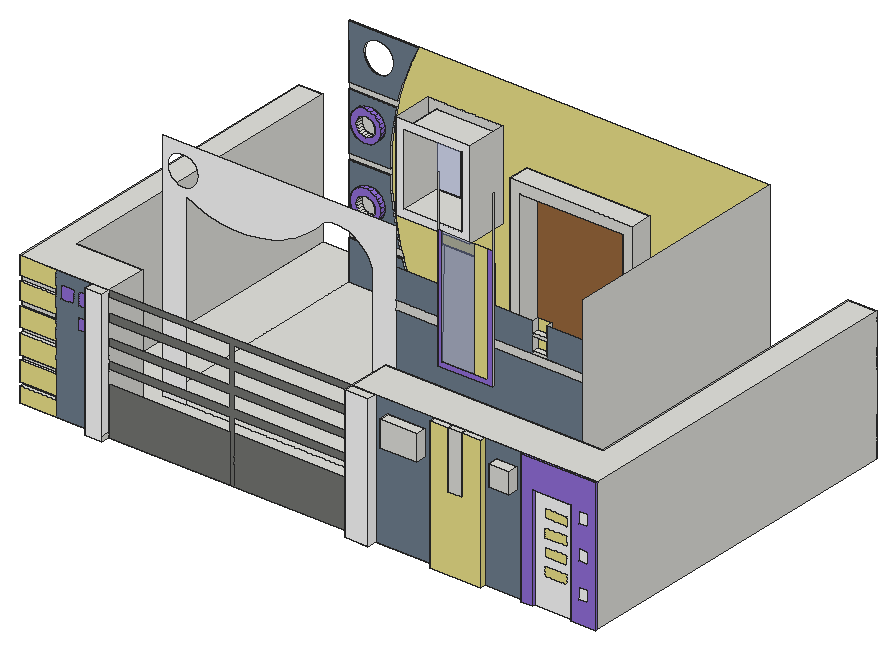
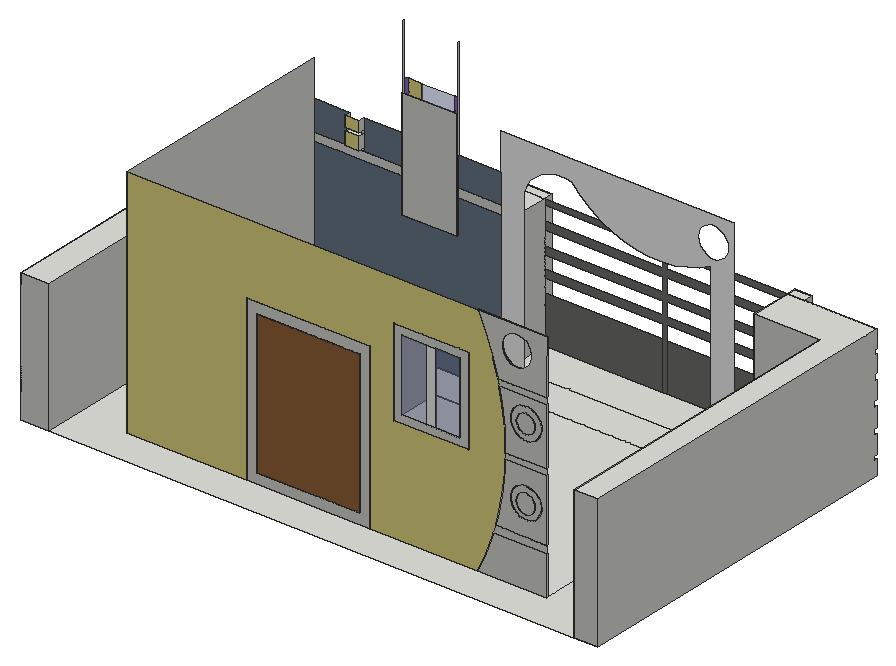
# SketchUp Ruby script. Lengths in inches.
U = 1.inch
M = Sketchup.active_model
def pt(a) = Geom::Point3d.new(a.map { |v| v * U })
def face(e, loops, mat)
  f = e.add_face(loops[0].map { |a| pt(a) })
  loops[1..].each { |l| e.add_face(l.map { |a| pt(a) }).erase! }
  f.material = f.back_material = mat if mat
  f
end
# faces: each face lists its corners as indices into pts; further lists are holes
def faces(e, pts, list, mat = nil) = list.each { |f| face(e, (f[0].is_a?(Array) ? f : [f]).map { |l| l.map { |i| pts[i] } }, mat) }
# xy, xz, yz: faces in a plane at the given z, y or x. An outline is a flat list of corners, or four numbers for a rectangle; further outlines are holes
def ring(l) = l.size == 4 ? [[l[0], l[1]], [l[2], l[1]], [l[2], l[3]], [l[0], l[3]]] : l.each_slice(2).to_a
def flat(e, list, mat, &to3) = list.each { |f| face(e, (f[0].is_a?(Array) ? f : [f]).map { |l| ring(l).map { |u, v| to3.(u, v) } }, mat) }
def xy(e, z, list, mat = nil) = flat(e, list, mat) { |x, y| [x, y, z] }
def xz(e, y, list, mat = nil) = flat(e, list, mat) { |x, z| [x, y, z] }
def yz(e, x, list, mat = nil) = flat(e, list, mat) { |y, z| [x, y, z] }
def lines(e, pts, list) = list.each { |a, b| e.add_line(pt(pts[a]), pt(pts[b])) }
# prism: a flat outline (further loops are holes) pulled along v
def prism(e, loops, v, mat = nil)
  f = face(e, loops, mat); d = Geom::Vector3d.new(v.map { |x| x * U })
  f.pushpull(f.normal.samedirection?(d) ? d.length : -d.length)
end
def box(e, o, s, mat = nil) = prism(e, [[o, [o[0] + s[0], o[1], o[2]], [o[0] + s[0], o[1] + s[1], o[2]], [o[0], o[1] + s[1], o[2]]]], [0, 0, s[2]], mat)
def at(x, y, z, deg = 0) = Geom::Transformation.translation(pt([x, y, z])) * Geom::Transformation.rotation(ORIGIN, Z_AXIS, deg.degrees)
def axes(o, x, y, z) = Geom::Transformation.new([*x, 0, *y, 0, *z, 0, *pt(o).to_a, 1])
def part(name) = M.definitions.add(name)
# library, detail: a bought-in or finely detailed component or shape, given as its bounding box
def library(name, o, s) = part(name).tap { |d| box(d.entities, o, s) }
def detail(e, o, s) = box(e.add_group.entities, o, s)
def put(e, d, t, mat = nil) = e.add_instance(d, t).tap { |i| i.material = mat if mat }
def group(e, t, mat = nil) = e.add_group.tap { |g| g.transformation = t; g.material = mat if mat }.entities
root = M.entities
M.materials.add("[0047_Khaki]").color = [240, 230, 140]
M.materials.add("[0111_SlateGray]").color = [112, 128, 144]
M.materials.add("[0115_MediumPurple]").color = [147, 112, 219]
M.materials.add("[0128_White]").color = [255, 255, 255]
M.materials.add("[Metal Seamed]").color = [118, 119, 115]
M.materials.add("[Translucent Glass Sky Reflection]").color = [126, 138, 183]
M.materials["[Translucent Glass Sky Reflection]"].alpha = 0.52
M.materials.add("[Wood Floor]").color = [155, 105, 61]
xy(root,0,[[36.78,0.6875,45.64,5.3125],[170.23,0.6875,182.3125,5.3125],[212.8,2.1875,238.66,5.3125],[258.03,3.6875,264.32,5.3125],[283.76,3.6875,296.5,5.3125],
  [0,5.3125,0,184,12.1,184,12.1,26.76,45.64,26.76,45.64,5.3125],[45.64,5.3125,170.23,26.76],[170.23,5.3125,170.23,26.76,282.06,26.76,282.06,184,296.5,184,296.5,5.3125],[[12.1,26.76,282.06,184],[40.75,45.625,256.75,165.625]],[40.75,45.625,40.75,164.9375,76.51,164.9375,76.51,165.625,131.6875,165.625,131.6875,154.6875,195,154.6875,195,165.625,256.75,165.625,256.75,45.625],
  [131.6875,154.6875,195,165.625],[40.75,164.9375,76.51,165.625]])
xy(root,5.41,[[137.1,154.6875,189.59,165.625]])
xy(root,7.86,[[0,5.3125,18.39,7.0625]])
xy(root,9.82,[[0,5.3125,18.39,7.0625]])
xy(root,19.55,[[0,5.3125,18.39,7.0625]])
xy(root,20.15,[[40.75,164.9375,68.39,165.625]])
xy(root,22.18,[[0,5.3125,18.39,7.0625]])
xy(root,24.17,[[40.75,164.9375,67.27,165.625]])
xy(root,32.3,[[0,5.3125,18.39,7.0625]])
xy(root,34.95,[[0,5.3125,18.39,7.0625]])
xy(root,38.3125,[[222.1,2.1875,228.92,5.3125]])
xy(root,44.42,[[0,5.3125,18.39,6.5]])
xy(root,47.25,[[0,5.3125,18.39,6.5]])
xy(root,47.92,[[188.84,0,207.78,5.3125]])
xy(root,49.69,[[244.53,0,255.09,5.3125]])
xy(root,53.625,[[264.32,3.6875,283.76,5.3125]],"[0115_MediumPurple]")
xy(root,53.875,[[81.125,144.5625,119.5625,165.625]])
xy(root,56.15,[[40.75,164.9375,62.41,165.625]])
xy(root,56.2,[[0,5.3125,18.39,6.5]])
xy(root,58.08,[[85.33,144.5625,115.36,165.625]])
xy(root,58.65,[[0,5.3125,18.39,6.5]])
xy(root,59.3125,[[40.75,164.9375,62.29,165.625]])
xy(root,60.25,[[244.53,0,255.09,5.3125]])
xy(root,61.11,[[188.84,0,207.78,5.3125]])
xy(root,64,[[182.75,44.5625,211.0625,45.625],[182.75,45.625,211.0625,45.9375]])
xy(root,67.8125,[[36.78,0.6875,45.64,5.3125],[170.23,0.6875,182.3125,5.3125],[212.8,2.1875,222.1,5.3125],[222.1,2.1875,228.92,5.3125],[228.92,2.1875,238.66,5.3125],
  [0,5.3125,45.64,5.3125,45.64,26.76,12.1,26.76,12.1,184,0,184],[170.23,5.3125,296.5,5.3125,296.5,184,282.06,184,282.06,26.76,170.23,26.76]])
xy(root,67.8125,[[258.03,3.6875,296.5,5.3125]],"[0115_MediumPurple]")
xy(root,78.59,[[137.1,154.6875,189.59,165.625]])
xy(root,84,[[131.6875,154.6875,195,165.625]])
xy(root,87.45,[[231.02,45.625,238.14,48.4375]])
xy(root,88.75,[[40.75,164.9375,65.47,165.625]])
xy(root,92.01,[[40.75,164.9375,66.2,165.625]])
xy(root,94.06,[[231.02,45.625,238.14,48.4375]])
xy(root,94.79,[[85.33,144.5625,115.36,165.625]])
xy(root,95.79,[[231.02,45.625,238.14,48.4375]])
xz(root,0,[[188.84,47.92,207.78,61.11],[244.53,49.69,255.09,60.25]])
xz(root,0.6875,[[36.78,0,45.64,67.8125],[170.23,0,182.3125,67.8125]],"[0128_White]")
xz(root,2.1875,[[222.1,38.3125,228.92,67.8125]])
xz(root,2.1875,[[212.8,0,238.66,0,238.66,67.8125,228.92,67.8125,228.92,38.3125,222.1,38.3125,222.1,67.8125,212.8,67.8125]],"[0047_Khaki]")
xz(root,3.6875,[[[258.03,0,264.32,0,264.32,53.625,283.76,53.625,283.76,0,296.5,0,296.5,67.8125,258.03,67.8125],[288.18,46.25,292.5,52.25],[288.18,29.0625,292.5,35.0625],[288.18,11.5,292.5,17.5]]],"[0115_MediumPurple]")
xz(root,3.6875,[[288.18,11.5,292.5,17.5],[288.18,29.0625,292.5,35.0625],[288.18,46.25,292.5,52.25]],"[0128_White]")
xz(root,5.3125,[[36.78,0,45.64,67.8125],[170.23,0,182.3125,67.8125],[212.8,0,212.8,67.8125,222.1,67.8125,222.1,38.3125,228.92,38.3125,228.92,67.8125,238.66,67.8125,238.66,0],[258.03,0,258.03,67.8125,296.5,67.8125,296.5,0,283.76,0,283.76,53.625,264.32,53.625,264.32,0],[222.1,38.3125,228.92,67.8125],
  [188.84,47.92,207.78,61.11],[244.53,49.69,255.09,60.25]])
xz(root,5.3125,[[0,0,18.39,7.86],[0,9.82,18.39,19.55],[269.1,14.74,280.41,19.43],[0,22.18,18.39,32.3],[269.1,23.68,280.41,28.37],
  [269.1,32.49,280.41,37.18],[0,34.95,18.39,44.42],[269.1,41.55,280.41,46.24],[0,47.25,18.39,56.2],[0,58.65,18.39,67.8125]],"[0047_Khaki]")
xz(root,5.3125,[[[18.39,0,36.78,67.8125],[20.96,55.08,27.39,61.52],[30.26,55.24,35.57,61.74],[30.26,44.17,35.95,49.85]],[[182.3125,0,212.8,67.8125],[188.84,47.92,207.78,61.11]],[[238.66,0,258.03,67.8125],[244.53,49.69,255.09,60.25]]],"[0111_SlateGray]")
xz(root,5.3125,[[30.26,44.17,35.95,49.85],[20.96,55.08,27.39,61.52],[30.26,55.24,35.57,61.74]],"[0115_MediumPurple]")
xz(root,5.3125,[[[264.32,0,283.76,53.625],[269.1,41.55,280.41,46.24],[269.1,32.49,280.41,37.18],[269.1,23.68,280.41,28.37],[269.1,14.74,280.41,19.43]]],"[0128_White]")
xz(root,5.3125,[[107.64,0,107.64,31.52,45.64,31.52,45.64,35.5,107.64,35.5,107.64,42.12,45.64,42.12,45.64,46.09,107.64,46.09,107.64,53.36,45.64,53.36,45.64,57.36,107.64,57.36,107.64,64.74,45.64,64.74,45.64,67.8125,170.23,67.8125,170.23,64.74,109.53,64.74,109.53,57.36,170.23,57.36,170.23,53.36,109.53,53.36,109.53,46.09,170.23,46.09,170.23,42.12,109.53,42.12,109.53,35.5,170.23,35.5,170.23,31.52,109.53,31.52,109.53,0],[45.64,0,107.64,24.54],[109.53,0,170.23,24.54]],"[Metal Seamed]")
xz(root,6.5,[[0,44.42,18.39,47.25],[0,56.2,18.39,58.65]])
xz(root,7.0625,[[0,7.86,18.39,9.82],[0,19.55,18.39,22.18],[0,32.3,18.39,34.95]])
xz(root,26.76,[[12.1,0,45.64,67.8125],[170.23,0,282.06,67.8125]])
xz(root,44.5625,[[201.68,66.53,208.37,66.53,208.5625,120,208.57,122.49,208.57,126.91,201.68,126.91]],"[0047_Khaki]")
xz(root,44.5625,[[182.75,64,211.0625,64,211.0625,126.91,208.57,126.91,208.57,120,208.5625,120,208.37,66.53,185.24,66.53,185.24,126.91,182.75,126.91]],"[0115_MediumPurple]")
xz(root,44.5625,[[185.24,66.53,201.68,126.91]],"[Translucent Glass Sky Reflection]")
xz(root,45.625,[[182.75,64,211.0625,120],[160.75,81.5,182.75,86],[211.0625,81.5,256.75,86],[231.02,86,238.14,87.45],[231.02,94.06,238.14,95.79]])
xz(root,45.625,[[160.75,0,256.75,0,256.75,81.5,211.0625,81.5,211.0625,64,182.75,64,182.75,81.5,160.75,81.5],[160.75,86,182.75,101.3125],[211.0625,86,231.02,101.3125],[238.14,86,256.75,101.3125]],"[0111_SlateGray]")
xz(root,45.625,[[[40.75,0,52.5,0,52.5,96,58.42,93.16,64.62,91.02,71.02,89.6,77.55,88.92,84.11,88.99,90.62,89.82,96.99,91.38,103.14,93.66,107.74,96,108.99,96.63,114.46,100.25,119.48,104.48,123.98,109.25,126.49,109.84,129.07,110.09,131.65,110.01,134.19,109.58,135.29,109.25,136.66,108.83,139.01,107.75,141.2,106.375,143.19,104.73,144.9375,102.83,146.42,100.72,147.62,98.43,148.5,96,148.5,0,160.75,0,160.75,120,40.75,120],[51.27,99.26,49.24,99.54,47.34,100.33,45.72,101.59,44.47,103.23,43.69,105.13,43.43,107.17,43.71,109.21,44.51,111.1,45.76,112.73,47.4,113.97,49.3,114.75,51.34,115.01,53.38,114.73,55.28,113.9375,56.9,112.68,58.14,111.04,58.92,109.14,59.18,107.1,58.91,105.0625,58.11,103.17,56.85,101.54,55.22,100.3,53.3125,99.52]]],"[0128_White]")
xz(root,45.9375,[[182.75,64,211.0625,120]])
xz(root,48.4375,[[231.02,87.45,238.14,94.06],[231.02,95.79,238.14,101.3125]],"[0047_Khaki]")
xz(root,144.5625,[[[81.125,53.875,119.5625,99],[85.33,58.08,115.36,94.79]]],"[0128_White]")
xz(root,154.6875,[[[131.6875,0,195,84],[137.1,5.41,189.59,78.59]]])
xz(root,162.1875,[[[50.59,32.03,52.66,32.05,54.66,32.6,56.45,33.65,57.9,35.13,58.92,36.93,59.4375,38.94,59.42,41.01,58.87,43.01,57.81,44.8,56.34,46.25,54.53,47.27,52.53,47.79,50.46,47.77,48.46,47.22,46.67,46.16,45.22,44.6875,44.2,42.88,43.68,40.88,43.7,38.81,44.25,36.81,45.3,35.02,46.78,33.57,48.59,32.55],[51.79,34.5625,50.53,34.73,49.36,35.21,48.35,35.99,47.57,37,47.09,38.17,46.92,39.4375,47.09,40.7,47.57,41.875,48.35,42.88,49.36,43.66,50.53,44.14,51.79,44.3125,53.06,44.14,54.23,43.66,55.24,42.88,56.02,41.875,56.5,40.7,56.67,39.4375,56.5,38.17,56.02,37,55.24,35.99,54.23,35.21,53.06,34.73]],[[50.59,68.53,52.66,68.55,54.66,69.1,56.45,70.15,57.9,71.63,58.92,73.43,59.4375,75.44,59.42,77.51,58.87,79.51,57.81,81.3,56.34,82.75,54.53,83.77,52.53,84.29,50.46,84.27,48.46,83.72,46.67,82.66,45.22,81.1875,44.2,79.38,43.68,77.38,43.7,75.31,44.25,73.31,45.3,71.52,46.78,70.07,48.59,69.05],[51.79,71.3125,50.53,71.48,49.36,71.96,48.35,72.74,47.57,73.75,47.09,74.92,46.92,76.1875,47.09,77.45,47.57,78.625,48.35,79.63,49.36,80.41,50.53,80.89,51.79,81.0625,53.06,80.89,54.23,80.41,55.24,79.63,56.02,78.625,56.5,77.45,56.67,76.1875,56.5,74.92,56.02,73.75,55.24,72.74,54.23,71.96,53.06,71.48]]],"[0115_MediumPurple]")
xz(root,164.9375,[[40.75,0,76.51,0,72.21,9.4375,68.66,19.18,68.39,20.15,40.75,20.15],[[40.75,24.17,67.27,24.17,65.875,29.17,63.87,39.34,62.67,49.64,62.41,56.15,40.75,56.15],[50.59,32.03,48.59,32.55,46.78,33.57,45.3,35.02,44.25,36.81,43.7,38.81,43.68,40.88,44.2,42.88,45.22,44.6875,46.67,46.16,48.46,47.22,50.46,47.77,52.53,47.79,54.53,47.27,56.34,46.25,57.81,44.8,58.87,43.01,59.42,41.01,59.4375,38.94,58.92,36.93,57.9,35.13,56.45,33.65,54.66,32.6,52.66,32.05]],[[40.75,59.3125,62.29,59.3125,62.26,60,62.67,70.36,63.87,80.66,65.47,88.75,40.75,88.75],[50.59,68.53,48.59,69.05,46.78,70.07,45.3,71.52,44.25,73.31,43.7,75.31,43.68,77.38,44.2,79.38,45.22,81.1875,46.67,82.66,48.46,83.72,50.46,84.27,52.53,84.29,54.53,83.77,56.34,82.75,57.81,81.3,58.87,79.51,59.42,77.51,59.4375,75.44,58.92,73.43,57.9,71.63,56.45,70.15,54.66,69.1,52.66,68.55]],[[40.75,92.01,66.2,92.01,68.66,100.82,72.21,110.5625,76.51,120,40.75,120],[55.29,100.3125,53.28,100.83,51.48,101.85,50,103.3,48.95,105.09,48.39,107.09,48.375,109.16,48.89,111.16,49.91,112.97,51.37,114.44,53.15,115.5,55.15,116.05,57.22,116.07,59.23,115.55,61.03,114.53,62.51,113.08,63.56,111.29,64.11,109.29,64.13,107.22,63.61,105.21,62.59,103.41,61.14,101.93,59.35,100.88,57.36,100.33]]],"[0111_SlateGray]")
xz(root,165.625,[[40.75,0,40.75,20.15,68.39,20.15,68.66,19.18,72.21,9.4375,76.51,0],[[131.6875,0,195,84],[137.1,5.41,189.59,78.59]],[40.75,20.15,40.75,24.17,67.27,24.17,68.39,20.15],[[40.75,24.17,40.75,56.15,62.41,56.15,62.67,49.64,63.87,39.34,65.875,29.17,67.27,24.17],[50.59,32.03,52.66,32.05,54.66,32.6,56.45,33.65,57.9,35.13,58.92,36.93,59.4375,38.94,59.42,41.01,58.87,43.01,57.81,44.8,56.34,46.25,54.53,47.27,52.53,47.79,50.46,47.77,48.46,47.22,46.67,46.16,45.22,44.6875,44.2,42.88,43.68,40.88,43.7,38.81,44.25,36.81,45.3,35.02,46.78,33.57,48.59,32.55]],[[50.59,32.03,48.59,32.55,46.78,33.57,45.3,35.02,44.25,36.81,43.7,38.81,43.68,40.88,44.2,42.88,45.22,44.6875,46.67,46.16,48.46,47.22,50.46,47.77,52.53,47.79,54.53,47.27,56.34,46.25,57.81,44.8,58.87,43.01,59.42,41.01,59.4375,38.94,58.92,36.93,57.9,35.13,56.45,33.65,54.66,32.6,52.66,32.05],[51.79,34.5625,53.06,34.73,54.23,35.21,55.24,35.99,56.02,37,56.5,38.17,56.67,39.4375,56.5,40.7,56.02,41.875,55.24,42.88,54.23,43.66,53.06,44.14,51.79,44.3125,50.53,44.14,49.36,43.66,48.35,42.88,47.57,41.875,47.09,40.7,46.92,39.4375,47.09,38.17,47.57,37,48.35,35.99,49.36,35.21,50.53,34.73]],
  [51.79,34.5625,50.53,34.73,49.36,35.21,48.35,35.99,47.57,37,47.09,38.17,46.92,39.4375,47.09,40.7,47.57,41.875,48.35,42.88,49.36,43.66,50.53,44.14,51.79,44.3125,53.06,44.14,54.23,43.66,55.24,42.88,56.02,41.875,56.5,40.7,56.67,39.4375,56.5,38.17,56.02,37,55.24,35.99,54.23,35.21,53.06,34.73],[[81.125,53.875,119.5625,99],[85.33,58.08,115.36,94.79]],[40.75,56.15,40.75,59.3125,62.29,59.3125,62.41,56.15],[[40.75,59.3125,40.75,88.75,65.47,88.75,63.87,80.66,62.67,70.36,62.26,60,62.29,59.3125],[50.59,68.53,52.66,68.55,54.66,69.1,56.45,70.15,57.9,71.63,58.92,73.43,59.4375,75.44,59.42,77.51,58.87,79.51,57.81,81.3,56.34,82.75,54.53,83.77,52.53,84.29,50.46,84.27,48.46,83.72,46.67,82.66,45.22,81.1875,44.2,79.38,43.68,77.38,43.7,75.31,44.25,73.31,45.3,71.52,46.78,70.07,48.59,69.05]],[[50.59,68.53,48.59,69.05,46.78,70.07,45.3,71.52,44.25,73.31,43.7,75.31,43.68,77.38,44.2,79.38,45.22,81.1875,46.67,82.66,48.46,83.72,50.46,84.27,52.53,84.29,54.53,83.77,56.34,82.75,57.81,81.3,58.87,79.51,59.42,77.51,59.4375,75.44,58.92,73.43,57.9,71.63,56.45,70.15,54.66,69.1,52.66,68.55],[51.79,71.3125,53.06,71.48,54.23,71.96,55.24,72.74,56.02,73.75,56.5,74.92,56.67,76.1875,56.5,77.45,56.02,78.625,55.24,79.63,54.23,80.41,53.06,80.89,51.79,81.0625,50.53,80.89,49.36,80.41,48.35,79.63,47.57,78.625,47.09,77.45,46.92,76.1875,47.09,74.92,47.57,73.75,48.35,72.74,49.36,71.96,50.53,71.48]],
  [51.79,71.3125,50.53,71.48,49.36,71.96,48.35,72.74,47.57,73.75,47.09,74.92,46.92,76.1875,47.09,77.45,47.57,78.625,48.35,79.63,49.36,80.41,50.53,80.89,51.79,81.0625,53.06,80.89,54.23,80.41,55.24,79.63,56.02,78.625,56.5,77.45,56.67,76.1875,56.5,74.92,56.02,73.75,55.24,72.74,54.23,71.96,53.06,71.48],[40.75,88.75,40.75,92.01,66.2,92.01,65.875,90.83,65.47,88.75],[[40.75,92.01,40.75,120,76.51,120,72.21,110.5625,68.66,100.82,66.2,92.01],[55.29,100.3125,57.36,100.33,59.35,100.88,61.14,101.93,62.59,103.41,63.61,105.21,64.13,107.22,64.11,109.29,63.56,111.29,62.51,113.08,61.03,114.53,59.23,115.55,57.22,116.07,55.15,116.05,53.15,115.5,51.37,114.44,49.91,112.97,48.89,111.16,48.375,109.16,48.39,107.09,48.95,105.09,50,103.3,51.48,101.85,53.28,100.83]]])
xz(root,165.625,[[[76.51,0,72.21,9.4375,68.66,19.18,68.39,20.15,67.27,24.17,65.875,29.17,63.87,39.34,62.67,49.64,62.41,56.15,62.29,59.3125,62.26,60,62.67,70.36,63.87,80.66,65.47,88.75,65.875,90.83,66.2,92.01,68.66,100.82,72.21,110.5625,76.51,120,256.75,120,256.75,0,195,0,195,84,131.6875,84,131.6875,0],[81.125,53.875,119.5625,99]]],"[0047_Khaki]")
xz(root,165.625,[[97.97,58.08,102.42,94.79]],"[0128_White]")
xz(root,165.625,[[85.33,58.08,97.97,94.79],[102.42,58.08,115.36,94.79]],"[Translucent Glass Sky Reflection]")
xz(root,165.625,[[137.1,5.41,189.59,78.59]],"[Wood Floor]")
xz(root,184,[[0,0,12.1,67.8125],[282.06,0,296.5,67.8125]])
yz(root,0,[[5.3125,0,5.3125,7.86,7.0625,7.86,7.0625,9.82,5.3125,9.82,5.3125,19.55,7.0625,19.55,7.0625,22.18,5.3125,22.18,5.3125,32.3,7.0625,32.3,7.0625,34.95,5.3125,34.95,5.3125,44.42,6.5,44.42,6.5,47.25,5.3125,47.25,5.3125,56.2,6.5,56.2,6.5,58.65,5.3125,58.65,5.3125,67.8125,184,67.8125,184,0]])
yz(root,12.1,[[26.76,0,184,67.8125]])
yz(root,18.39,[[5.3125,7.86,7.0625,9.82],[5.3125,19.55,7.0625,22.18],[5.3125,32.3,7.0625,34.95],[5.3125,44.42,6.5,47.25],[5.3125,56.2,6.5,58.65]])
yz(root,36.78,[[0.6875,0,5.3125,67.8125]])
yz(root,40.75,[[164.9375,0,165.625,20.15],[164.9375,24.17,165.625,56.15],[164.9375,59.3125,165.625,88.75],[164.9375,92.01,165.625,111.01]])
yz(root,45.64,[[0.6875,0,5.3125,2.5],[5.3125,0,26.76,67.8125]])
yz(root,45.64,[[0.6875,2.5,5.3125,67.8125]],"[0128_White]")
yz(root,81.125,[[144.5625,53.875,165.625,99]])
yz(root,85.33,[[144.5625,58.08,165.625,94.79]])
yz(root,115.36,[[144.5625,58.08,165.625,94.79]])
yz(root,119.5625,[[144.5625,53.875,165.625,99]])
yz(root,131.6875,[[154.6875,0,165.625,84]])
yz(root,137.1,[[154.6875,5.41,165.625,78.59]])
yz(root,170.23,[[0.6875,0,5.3125,67.8125],[5.3125,0,26.76,67.8125]])
yz(root,182.3125,[[0.6875,0,5.3125,67.8125]],"[0128_White]")
yz(root,182.75,[[44.5625,64,45.625,152.8125],[45.625,64,45.9375,120]])
yz(root,185.24,[[44.5625,66.53,45.625,120,44.5625,120]])
yz(root,188.84,[[0,47.92,5.3125,61.11]])
yz(root,189.59,[[154.6875,5.41,165.625,78.59]])
yz(root,195,[[154.6875,0,165.625,84]])
yz(root,207.78,[[0,47.92,5.3125,61.11]])
yz(root,211.0625,[[44.5625,64,45.625,152.8125],[45.625,64,45.9375,120]])
yz(root,212.8,[[2.1875,0,5.3125,67.8125]])
yz(root,222.1,[[2.1875,38.3125,5.3125,67.8125]])
yz(root,228.92,[[2.1875,38.3125,5.3125,67.8125]])
yz(root,231.02,[[45.625,87.45,48.4375,94.06],[45.625,95.79,48.4375,101.3125]])
yz(root,238.14,[[45.625,87.45,48.4375,94.06],[45.625,95.79,48.4375,101.3125]])
yz(root,238.66,[[2.1875,0,5.3125,67.8125]],"[0047_Khaki]")
yz(root,244.53,[[0,49.69,5.3125,60.25]])
yz(root,255.09,[[0,49.69,5.3125,60.25]])
yz(root,256.75,[[45.625,0,165.625,120]])
yz(root,258.03,[[3.6875,0,5.3125,67.8125]],"[0115_MediumPurple]")
yz(root,264.32,[[3.6875,0,5.3125,53.625]],"[0115_MediumPurple]")
yz(root,282.06,[[26.76,0,184,67.8125]])
yz(root,283.76,[[3.6875,0,5.3125,53.625]],"[0115_MediumPurple]")
yz(root,296.5,[[5.3125,0,184,67.8125]])
yz(root,296.5,[[3.6875,0,5.3125,67.8125]],"[0115_MediumPurple]")
p = [[76.51,165.625,0],[72.21,165.625,9.4375],[72.21,164.9375,9.4375],[76.51,164.9375,0],[68.66,165.625,19.18],[68.66,164.9375,19.18],
  [68.39,165.625,20.15],[68.39,164.9375,20.15],[67.27,165.625,24.17],[65.875,165.625,29.17],[65.875,164.9375,29.17],[67.27,164.9375,24.17],
  [63.87,165.625,39.34],[63.87,164.9375,39.34],[48.59,162.1875,32.55],[48.59,164.9375,32.55],[50.59,164.9375,32.03],[50.59,162.1875,32.03],
  [52.66,164.9375,32.05],[52.66,162.1875,32.05],[54.66,164.9375,32.6],[54.66,162.1875,32.6],[48.59,165.625,32.55],[50.59,165.625,32.03],
  [52.66,165.625,32.05],[54.66,165.625,32.6],[46.78,162.1875,33.57],[46.78,164.9375,33.57],[46.78,165.625,33.57],[56.45,164.9375,33.65],
  [56.45,162.1875,33.65],[56.45,165.625,33.65],[45.3,162.1875,35.02],[45.3,164.9375,35.02],[45.3,165.625,35.02],[57.9,164.9375,35.13],
  [57.9,162.1875,35.13],[57.9,165.625,35.13],[51.79,165.625,34.5625],[50.53,165.625,34.73],[50.53,162.1875,34.73],[51.79,162.1875,34.5625],
  [53.06,165.625,34.73],[53.06,162.1875,34.73],[49.36,165.625,35.21],[49.36,162.1875,35.21],[54.23,165.625,35.21],[54.23,162.1875,35.21],
  [44.25,162.1875,36.81],[44.25,164.9375,36.81],[44.25,165.625,36.81],[58.92,164.9375,36.93],[58.92,162.1875,36.93],[58.92,165.625,36.93],
  [48.35,165.625,35.99],[48.35,162.1875,35.99],[55.24,165.625,35.99],[55.24,162.1875,35.99],[47.57,165.625,37],[47.57,162.1875,37],
  [56.02,165.625,37],[56.02,162.1875,37],[43.7,162.1875,38.81],[43.7,164.9375,38.81],[43.7,165.625,38.81],[59.4375,164.9375,38.94],
  [59.4375,162.1875,38.94],[59.4375,165.625,38.94],[47.09,165.625,38.17],[47.09,162.1875,38.17],[56.5,165.625,38.17],[56.5,162.1875,38.17],
  [46.92,165.625,39.4375],[46.92,162.1875,39.4375],[56.67,165.625,39.4375],[56.67,162.1875,39.4375],[43.68,162.1875,40.88],[43.68,164.9375,40.88],
  [43.68,165.625,40.88],[59.42,164.9375,41.01],[59.42,162.1875,41.01],[59.42,165.625,41.01],[62.67,165.625,49.64],[62.67,164.9375,49.64],
  [47.09,165.625,40.7],[47.09,162.1875,40.7],[56.5,165.625,40.7],[56.5,162.1875,40.7],[47.57,165.625,41.875],[47.57,162.1875,41.875],
  [56.02,165.625,41.875],[56.02,162.1875,41.875],[44.2,162.1875,42.88],[44.2,164.9375,42.88],[44.2,165.625,42.88],[58.87,164.9375,43.01],
  [58.87,162.1875,43.01],[58.87,165.625,43.01],[48.35,165.625,42.88],[48.35,162.1875,42.88],[55.24,165.625,42.88],[55.24,162.1875,42.88],
  [45.22,162.1875,44.6875],[45.22,164.9375,44.6875],[49.36,165.625,43.66],[49.36,162.1875,43.66],[54.23,165.625,43.66],[54.23,162.1875,43.66],
  [45.22,165.625,44.6875],[57.81,164.9375,44.8],[57.81,162.1875,44.8],[57.81,165.625,44.8],[50.53,165.625,44.14],[50.53,162.1875,44.14],
  [53.06,165.625,44.14],[53.06,162.1875,44.14],[51.79,165.625,44.3125],[51.79,162.1875,44.3125],[46.67,162.1875,46.16],[46.67,164.9375,46.16],
  [46.67,165.625,46.16],[56.34,164.9375,46.25],[56.34,162.1875,46.25],[56.34,165.625,46.25],[48.46,162.1875,47.22],[48.46,164.9375,47.22],
  [54.53,164.9375,47.27],[54.53,162.1875,47.27],[48.46,165.625,47.22],[54.53,165.625,47.27],[50.46,162.1875,47.77],[50.46,164.9375,47.77],
  [50.46,165.625,47.77],[52.53,164.9375,47.79],[52.53,162.1875,47.79],[52.53,165.625,47.79],[62.41,165.625,56.15],[62.41,164.9375,56.15],
  [62.29,165.625,59.3125],[62.26,165.625,60],[62.26,164.9375,60],[62.29,164.9375,59.3125],[62.67,165.625,70.36],[62.67,164.9375,70.36],
  [48.59,162.1875,69.05],[48.59,164.9375,69.05],[50.59,164.9375,68.53],[50.59,162.1875,68.53],[52.66,164.9375,68.55],[52.66,162.1875,68.55],
  [54.66,164.9375,69.1],[54.66,162.1875,69.1],[48.59,165.625,69.05],[50.59,165.625,68.53],[52.66,165.625,68.55],[54.66,165.625,69.1],
  [46.78,162.1875,70.07],[46.78,164.9375,70.07],[46.78,165.625,70.07],[56.45,164.9375,70.15],[56.45,162.1875,70.15],[56.45,165.625,70.15],
  [45.3,162.1875,71.52],[45.3,164.9375,71.52],[45.3,165.625,71.52],[57.9,164.9375,71.63],[57.9,162.1875,71.63],[57.9,165.625,71.63],
  [63.87,165.625,80.66],[63.87,164.9375,80.66],[51.79,165.625,71.3125],[50.53,165.625,71.48],[50.53,162.1875,71.48],[51.79,162.1875,71.3125],
  [53.06,165.625,71.48],[53.06,162.1875,71.48],[44.25,162.1875,73.31],[44.25,164.9375,73.31],[49.36,165.625,71.96],[49.36,162.1875,71.96],
  [54.23,165.625,71.96],[54.23,162.1875,71.96],[44.25,165.625,73.31],[58.92,164.9375,73.43],[58.92,162.1875,73.43],[58.92,165.625,73.43],
  [48.35,165.625,72.74],[48.35,162.1875,72.74],[55.24,165.625,72.74],[55.24,162.1875,72.74],[47.57,165.625,73.75],[47.57,162.1875,73.75],
  [56.02,165.625,73.75],[56.02,162.1875,73.75],[43.7,162.1875,75.31],[43.7,164.9375,75.31],[43.7,165.625,75.31],[59.4375,164.9375,75.44],
  [59.4375,162.1875,75.44],[59.4375,165.625,75.44],[47.09,165.625,74.92],[47.09,162.1875,74.92],[56.5,165.625,74.92],[56.5,162.1875,74.92],
  [46.92,165.625,76.1875],[46.92,162.1875,76.1875],[56.67,165.625,76.1875],[56.67,162.1875,76.1875],[43.68,162.1875,77.38],[43.68,164.9375,77.38],
  [43.68,165.625,77.38],[59.42,164.9375,77.51],[59.42,162.1875,77.51],[59.42,165.625,77.51],[47.09,165.625,77.45],[47.09,162.1875,77.45],
  [56.5,165.625,77.45],[56.5,162.1875,77.45],[44.2,162.1875,79.38],[44.2,164.9375,79.38],[47.57,165.625,78.625],[47.57,162.1875,78.625],
  [56.02,165.625,78.625],[56.02,162.1875,78.625],[44.2,165.625,79.38],[58.87,164.9375,79.51],[58.87,162.1875,79.51],[58.87,165.625,79.51],
  [48.35,165.625,79.63],[48.35,162.1875,79.63],[55.24,165.625,79.63],[55.24,162.1875,79.63],[45.22,162.1875,81.1875],[45.22,164.9375,81.1875],
  [45.22,165.625,81.1875],[57.81,164.9375,81.3],[57.81,162.1875,81.3],[57.81,165.625,81.3],[49.36,165.625,80.41],[49.36,162.1875,80.41],
  [54.23,165.625,80.41],[54.23,162.1875,80.41],[50.53,165.625,80.89],[50.53,162.1875,80.89],[53.06,165.625,80.89],[53.06,162.1875,80.89],
  [65.47,165.625,88.75],[65.47,164.9375,88.75],[51.79,165.625,81.0625],[51.79,162.1875,81.0625],[46.67,162.1875,82.66],[46.67,164.9375,82.66],
  [46.67,165.625,82.66],[56.34,164.9375,82.75],[56.34,162.1875,82.75],[56.34,165.625,82.75],[48.46,162.1875,83.72],[48.46,164.9375,83.72],
  [54.53,164.9375,83.77],[54.53,162.1875,83.77],[48.46,165.625,83.72],[54.53,165.625,83.77],[50.46,162.1875,84.27],[50.46,164.9375,84.27],
  [50.46,165.625,84.27],[52.53,164.9375,84.29],[52.53,162.1875,84.29],[52.53,165.625,84.29],[66.2,165.625,92.01],[68.66,165.625,100.82],
  [68.66,164.9375,100.82],[66.2,164.9375,92.01],[185.24,44.5625,66.53],[208.57,45.52,66.53],[208.57,45.625,120]]
faces(root,p,[[0,1,2,3],[1,4,5,2],[4,6,7,5],[8,9,10,11],[9,12,13,10],[22,23,16,15],[23,24,18,16],[24,25,20,18],
  [28,22,15,27],[25,31,29,20],[34,28,27,33],[31,37,35,29],[38,39,40,41],[42,38,41,43],[39,44,45,40],[46,42,43,47],
  [50,34,33,49],[37,53,51,35],[44,54,55,45],[56,46,47,57],[54,58,59,55],[60,56,57,61],[64,50,49,63],[53,67,65,51],
  [58,68,69,59],[70,60,61,71],[68,72,73,69],[74,70,71,75],[78,64,63,77],[67,81,79,65],[12,82,83,13],[72,84,85,73],
  [86,74,75,87],[84,88,89,85],[90,86,87,91],[94,78,77,93],[81,97,95,79],[88,98,99,89],[100,90,91,101],[98,104,105,99],
  [106,100,101,107],[108,94,93,103],[97,111,109,95],[104,112,113,105],[114,106,107,115],[112,116,117,113],[116,114,115,117],[120,108,103,119],
  [111,123,121,109],[128,120,119,125],[123,129,126,121],[132,128,125,131],[129,135,133,126],[135,132,131,133],[82,136,137,83],[138,139,140,141],
  [139,142,143,140],[152,153,146,145],[153,154,148,146],[154,155,150,148],[158,152,145,157],[155,161,159,150],[164,158,157,163],[161,167,165,159],
  [142,168,169,143],[170,171,172,173],[174,170,173,175],[171,178,179,172],[180,174,175,181],[182,164,163,177],[167,185,183,165],[178,186,187,179],
  [188,180,181,189],[186,190,191,187],[192,188,189,193],[196,182,177,195],[185,199,197,183],[190,200,201,191],[202,192,193,203],[200,204,205,201],
  [206,202,203,207],[210,196,195,209],[199,213,211,197],[204,214,215,205],[216,206,207,217],[214,220,221,215],[222,216,217,223],[224,210,209,219],
  [213,227,225,211],[220,228,229,221],[230,222,223,231],[234,224,219,233],[227,237,235,225],[228,238,239,229],[240,230,231,241],[238,242,243,239],
  [244,240,241,245],[168,246,247,169],[242,248,249,243],[248,244,245,249],[252,234,233,251],[237,255,253,235],[260,252,251,257],[255,261,258,253],
  [264,260,257,263],[261,267,265,258],[267,264,263,265],[268,269,270,271]])
faces(root,p,[[14,15,16,17],[17,16,18,19],[19,18,20,21],[26,27,15,14],[21,20,29,30],[32,33,27,26],[30,29,35,36],[48,49,33,32],
  [36,35,51,52],[62,63,49,48],[52,51,65,66],[76,77,63,62],[66,65,79,80],[92,93,77,76],[80,79,95,96],[102,103,93,92],
  [96,95,109,110],[118,119,103,102],[110,109,121,122],[124,125,119,118],[122,121,126,127],[130,131,125,124],[127,126,133,134],[134,133,131,130],
  [144,145,146,147],[147,146,148,149],[149,148,150,151],[156,157,145,144],[151,150,159,160],[162,163,157,156],[160,159,165,166],[176,177,163,162],
  [166,165,183,184],[194,195,177,176],[184,183,197,198],[208,209,195,194],[198,197,211,212],[218,219,209,208],[212,211,225,226],[232,233,219,218],
  [226,225,235,236],[250,251,233,232],[236,235,253,254],[256,257,251,250],[254,253,258,259],[262,263,257,256],[259,258,265,266],[266,265,263,262]],"[0115_MediumPurple]")
lines(root,p,[[272,273],[274,273]])
